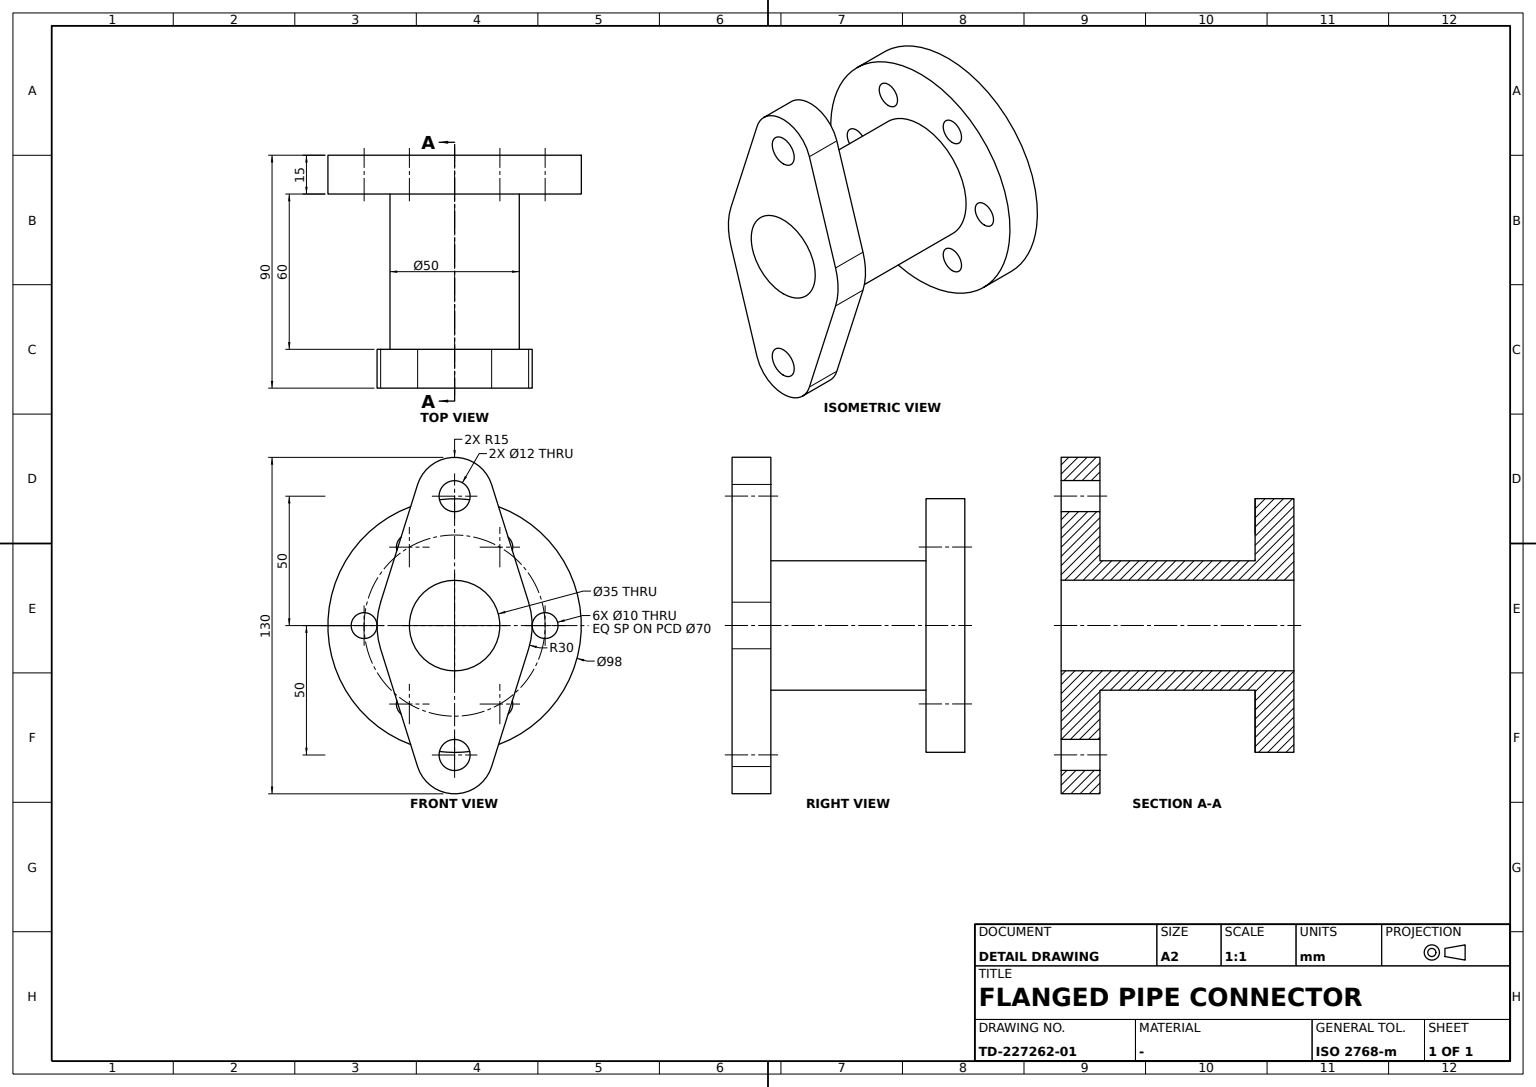
ISO-10303-21;
HEADER;
FILE_DESCRIPTION((''),'2;1');
FILE_NAME('','',(''),(''),'','','');
FILE_SCHEMA(('AUTOMOTIVE_DESIGN'));
ENDSEC;
DATA;
#1=APPLICATION_CONTEXT('');
#2=PRODUCT_CONTEXT('',#1,'mechanical');
#3=PRODUCT('','','',(#2));
#4=PRODUCT_DEFINITION_FORMATION('','',#3);
#5=PRODUCT_DEFINITION_CONTEXT('',#1,'design');
#6=PRODUCT_DEFINITION('','',#4,#5);
#7=PRODUCT_DEFINITION_SHAPE('','',#6);
#8=(LENGTH_UNIT()NAMED_UNIT(*)SI_UNIT(.MILLI.,.METRE.));
#9=(NAMED_UNIT(*)PLANE_ANGLE_UNIT()SI_UNIT($,.RADIAN.));
#10=(NAMED_UNIT(*)SI_UNIT($,.STERADIAN.)SOLID_ANGLE_UNIT());
#11=UNCERTAINTY_MEASURE_WITH_UNIT(LENGTH_MEASURE(0.005),#8,'distance_accuracy_value','');
#12=(GEOMETRIC_REPRESENTATION_CONTEXT(3)GLOBAL_UNCERTAINTY_ASSIGNED_CONTEXT((#11))GLOBAL_UNIT_ASSIGNED_CONTEXT((#8,#9,#10))REPRESENTATION_CONTEXT('',''));
#13=CARTESIAN_POINT('',(15.,0.,-25.));
#14=VERTEX_POINT('',#13);
#15=CARTESIAN_POINT('',(15.,0.,0.));
#16=DIRECTION('',(1.,0.,0.));
#17=DIRECTION('',(0.,0.,-1.));
#18=AXIS2_PLACEMENT_3D('',#15,#16,#17);
#19=CIRCLE('',#18,25.);
#20=EDGE_CURVE('',#14,#14,#19,.T.);
#21=ORIENTED_EDGE('',*,*,#20,.T.);
#22=EDGE_LOOP('',(#21));
#23=FACE_BOUND('',#22,.T.);
#24=CARTESIAN_POINT('',(75.,0.,-25.));
#25=VERTEX_POINT('',#24);
#26=CARTESIAN_POINT('',(75.,0.,0.));
#27=AXIS2_PLACEMENT_3D('',#26,#16,#17);
#28=CIRCLE('',#27,25.);
#29=EDGE_CURVE('',#25,#25,#28,.T.);
#30=ORIENTED_EDGE('',*,*,#29,.F.);
#31=EDGE_LOOP('',(#30));
#32=FACE_BOUND('',#31,.T.);
#33=CARTESIAN_POINT('',(45.,0.,0.));
#34=DIRECTION('',(0.,1.,0.));
#35=AXIS2_PLACEMENT_3D('',#33,#16,#34);
#36=CYLINDRICAL_SURFACE('',#35,25.);
#37=ADVANCED_FACE('',(#23,#32),#36,.T.);
#38=CARTESIAN_POINT('',(90.,0.,-56.));
#39=VERTEX_POINT('',#38);
#40=CARTESIAN_POINT('',(90.,0.,-50.));
#41=AXIS2_PLACEMENT_3D('',#40,#16,#17);
#42=CIRCLE('',#41,6.);
#43=EDGE_CURVE('',#39,#39,#42,.T.);
#44=ORIENTED_EDGE('',*,*,#43,.T.);
#45=EDGE_LOOP('',(#44));
#46=FACE_BOUND('',#45,.T.);
#47=CARTESIAN_POINT('',(75.,0.,-56.));
#48=VERTEX_POINT('',#47);
#49=CARTESIAN_POINT('',(75.,0.,-50.));
#50=AXIS2_PLACEMENT_3D('',#49,#16,#17);
#51=CIRCLE('',#50,6.);
#52=EDGE_CURVE('',#48,#48,#51,.T.);
#53=ORIENTED_EDGE('',*,*,#52,.F.);
#54=EDGE_LOOP('',(#53));
#55=FACE_BOUND('',#54,.T.);
#56=CARTESIAN_POINT('',(82.5,0.,-50.));
#57=AXIS2_PLACEMENT_3D('',#56,#16,#34);
#58=CYLINDRICAL_SURFACE('',#57,6.);
#59=ADVANCED_FACE('',(#46,#55),#58,.F.);
#60=CARTESIAN_POINT('',(0.,17.5,-35.310889));
#61=VERTEX_POINT('',#60);
#62=CARTESIAN_POINT('',(0.,17.5,-30.310889));
#63=AXIS2_PLACEMENT_3D('',#62,#16,#17);
#64=CIRCLE('',#63,5.);
#65=EDGE_CURVE('',#61,#61,#64,.T.);
#66=ORIENTED_EDGE('',*,*,#65,.F.);
#67=EDGE_LOOP('',(#66));
#68=FACE_BOUND('',#67,.T.);
#69=CARTESIAN_POINT('',(15.,17.5,-35.310889));
#70=VERTEX_POINT('',#69);
#71=CARTESIAN_POINT('',(15.,17.5,-30.310889));
#72=AXIS2_PLACEMENT_3D('',#71,#16,#17);
#73=CIRCLE('',#72,5.);
#74=EDGE_CURVE('',#70,#70,#73,.T.);
#75=ORIENTED_EDGE('',*,*,#74,.T.);
#76=EDGE_LOOP('',(#75));
#77=FACE_BOUND('',#76,.T.);
#78=CARTESIAN_POINT('',(7.5,17.5,-30.310889));
#79=AXIS2_PLACEMENT_3D('',#78,#16,#34);
#80=CYLINDRICAL_SURFACE('',#79,5.);
#81=ADVANCED_FACE('',(#68,#77),#80,.F.);
#82=CARTESIAN_POINT('',(15.,0.,-49.));
#83=VERTEX_POINT('',#82);
#84=CIRCLE('',#18,49.);
#85=EDGE_CURVE('',#83,#83,#84,.T.);
#86=ORIENTED_EDGE('',*,*,#85,.F.);
#87=EDGE_LOOP('',(#86));
#88=FACE_BOUND('',#87,.T.);
#89=CARTESIAN_POINT('',(0.,0.,-49.));
#90=VERTEX_POINT('',#89);
#91=CARTESIAN_POINT('',(0.,0.,0.));
#92=AXIS2_PLACEMENT_3D('',#91,#16,#17);
#93=CIRCLE('',#92,49.);
#94=EDGE_CURVE('',#90,#90,#93,.T.);
#95=ORIENTED_EDGE('',*,*,#94,.T.);
#96=EDGE_LOOP('',(#95));
#97=FACE_BOUND('',#96,.T.);
#98=CARTESIAN_POINT('',(7.5,0.,0.));
#99=AXIS2_PLACEMENT_3D('',#98,#16,#34);
#100=CYLINDRICAL_SURFACE('',#99,49.);
#101=ADVANCED_FACE('',(#88,#97),#100,.T.);
#102=CARTESIAN_POINT('',(75.,-28.618176,9.));
#103=VERTEX_POINT('',#102);
#104=CARTESIAN_POINT('',(90.,-28.618176,9.));
#105=VERTEX_POINT('',#104);
#106=CARTESIAN_POINT('',(82.5,-28.618176,9.));
#107=VECTOR('',#16,1000.);
#108=LINE('',#106,#107);
#109=EDGE_CURVE('',#103,#105,#108,.T.);
#110=ORIENTED_EDGE('',*,*,#109,.T.);
#111=CARTESIAN_POINT('',(90.,-14.309088,54.5));
#112=VERTEX_POINT('',#111);
#113=DIRECTION('',(0.,0.3,0.953939201));
#114=VECTOR('',#113,1000.);
#115=LINE('',#104,#114);
#116=EDGE_CURVE('',#105,#112,#115,.T.);
#117=ORIENTED_EDGE('',*,*,#116,.T.);
#118=CARTESIAN_POINT('',(75.,-14.309088,54.5));
#119=VERTEX_POINT('',#118);
#120=CARTESIAN_POINT('',(82.5,-14.309088,54.5));
#121=LINE('',#120,#107);
#122=EDGE_CURVE('',#119,#112,#121,.T.);
#123=ORIENTED_EDGE('',*,*,#122,.F.);
#124=LINE('',#102,#114);
#125=EDGE_CURVE('',#103,#119,#124,.T.);
#126=ORIENTED_EDGE('',*,*,#125,.F.);
#127=EDGE_LOOP('',(#110,#117,#123,#126));
#128=FACE_BOUND('',#127,.T.);
#129=DIRECTION('',(0.,0.953939201,-0.3));
#130=AXIS2_PLACEMENT_3D('',#102,#129,#113);
#131=PLANE('',#130);
#132=ADVANCED_FACE('',(#128),#131,.F.);
#133=CARTESIAN_POINT('',(75.,14.309088,-54.5));
#134=VERTEX_POINT('',#133);
#135=CARTESIAN_POINT('',(75.,28.618176,-9.));
#136=VERTEX_POINT('',#135);
#137=LINE('',#135,#114);
#138=EDGE_CURVE('',#134,#136,#137,.T.);
#139=ORIENTED_EDGE('',*,*,#138,.T.);
#140=CARTESIAN_POINT('',(90.,28.618176,-9.));
#141=VERTEX_POINT('',#140);
#142=CARTESIAN_POINT('',(82.5,28.618176,-9.));
#143=LINE('',#142,#107);
#144=EDGE_CURVE('',#136,#141,#143,.T.);
#145=ORIENTED_EDGE('',*,*,#144,.T.);
#146=CARTESIAN_POINT('',(90.,14.309088,-54.5));
#147=VERTEX_POINT('',#146);
#148=LINE('',#140,#114);
#149=EDGE_CURVE('',#147,#141,#148,.T.);
#150=ORIENTED_EDGE('',*,*,#149,.F.);
#151=CARTESIAN_POINT('',(82.5,14.309088,-54.5));
#152=LINE('',#151,#107);
#153=EDGE_CURVE('',#134,#147,#152,.T.);
#154=ORIENTED_EDGE('',*,*,#153,.F.);
#155=EDGE_LOOP('',(#139,#145,#150,#154));
#156=FACE_BOUND('',#155,.T.);
#157=AXIS2_PLACEMENT_3D('',#133,#129,#113);
#158=PLANE('',#157);
#159=ADVANCED_FACE('',(#156),#158,.T.);
#160=CARTESIAN_POINT('',(90.,14.309088,54.5));
#161=VERTEX_POINT('',#160);
#162=CARTESIAN_POINT('',(90.,28.618176,9.));
#163=VERTEX_POINT('',#162);
#164=DIRECTION('',(0.,0.3,-0.953939201));
#165=VECTOR('',#164,1000.);
#166=LINE('',#162,#165);
#167=EDGE_CURVE('',#161,#163,#166,.T.);
#168=ORIENTED_EDGE('',*,*,#167,.T.);
#169=CARTESIAN_POINT('',(75.,28.618176,9.));
#170=VERTEX_POINT('',#169);
#171=CARTESIAN_POINT('',(82.5,28.618176,9.));
#172=LINE('',#171,#107);
#173=EDGE_CURVE('',#170,#163,#172,.T.);
#174=ORIENTED_EDGE('',*,*,#173,.F.);
#175=CARTESIAN_POINT('',(75.,14.309088,54.5));
#176=VERTEX_POINT('',#175);
#177=LINE('',#169,#165);
#178=EDGE_CURVE('',#176,#170,#177,.T.);
#179=ORIENTED_EDGE('',*,*,#178,.F.);
#180=CARTESIAN_POINT('',(82.5,14.309088,54.5));
#181=LINE('',#180,#107);
#182=EDGE_CURVE('',#176,#161,#181,.T.);
#183=ORIENTED_EDGE('',*,*,#182,.T.);
#184=EDGE_LOOP('',(#168,#174,#179,#183));
#185=FACE_BOUND('',#184,.T.);
#186=DIRECTION('',(0.,-0.953939201,-0.3));
#187=AXIS2_PLACEMENT_3D('',#175,#186,#164);
#188=PLANE('',#187);
#189=ADVANCED_FACE('',(#185),#188,.F.);
#190=CARTESIAN_POINT('',(15.,-17.5,-35.310889));
#191=VERTEX_POINT('',#190);
#192=CARTESIAN_POINT('',(15.,-17.5,-30.310889));
#193=AXIS2_PLACEMENT_3D('',#192,#16,#17);
#194=CIRCLE('',#193,5.);
#195=EDGE_CURVE('',#191,#191,#194,.T.);
#196=ORIENTED_EDGE('',*,*,#195,.T.);
#197=EDGE_LOOP('',(#196));
#198=FACE_BOUND('',#197,.T.);
#199=CARTESIAN_POINT('',(0.,-17.5,-35.310889));
#200=VERTEX_POINT('',#199);
#201=CARTESIAN_POINT('',(0.,-17.5,-30.310889));
#202=AXIS2_PLACEMENT_3D('',#201,#16,#17);
#203=CIRCLE('',#202,5.);
#204=EDGE_CURVE('',#200,#200,#203,.T.);
#205=ORIENTED_EDGE('',*,*,#204,.F.);
#206=EDGE_LOOP('',(#205));
#207=FACE_BOUND('',#206,.T.);
#208=CARTESIAN_POINT('',(7.5,-17.5,-30.310889));
#209=AXIS2_PLACEMENT_3D('',#208,#16,#34);
#210=CYLINDRICAL_SURFACE('',#209,5.);
#211=ADVANCED_FACE('',(#198,#207),#210,.F.);
#212=CARTESIAN_POINT('',(90.,0.,-17.5));
#213=VERTEX_POINT('',#212);
#214=CARTESIAN_POINT('',(90.,0.,0.));
#215=AXIS2_PLACEMENT_3D('',#214,#16,#17);
#216=CIRCLE('',#215,17.5);
#217=EDGE_CURVE('',#213,#213,#216,.T.);
#218=ORIENTED_EDGE('',*,*,#217,.T.);
#219=EDGE_LOOP('',(#218));
#220=FACE_BOUND('',#219,.T.);
#221=CARTESIAN_POINT('',(0.,0.,-17.5));
#222=VERTEX_POINT('',#221);
#223=CIRCLE('',#92,17.5);
#224=EDGE_CURVE('',#222,#222,#223,.T.);
#225=ORIENTED_EDGE('',*,*,#224,.F.);
#226=EDGE_LOOP('',(#225));
#227=FACE_BOUND('',#226,.T.);
#228=CARTESIAN_POINT('',(44.34,0.,0.));
#229=AXIS2_PLACEMENT_3D('',#228,#16,#34);
#230=CYLINDRICAL_SURFACE('',#229,17.5);
#231=ADVANCED_FACE('',(#220,#227),#230,.F.);
#232=CARTESIAN_POINT('',(75.,0.,44.));
#233=VERTEX_POINT('',#232);
#234=CARTESIAN_POINT('',(75.,0.,50.));
#235=AXIS2_PLACEMENT_3D('',#234,#16,#17);
#236=CIRCLE('',#235,6.);
#237=EDGE_CURVE('',#233,#233,#236,.T.);
#238=ORIENTED_EDGE('',*,*,#237,.T.);
#239=EDGE_LOOP('',(#238));
#240=FACE_BOUND('',#239,.T.);
#241=ORIENTED_EDGE('',*,*,#125,.T.);
#242=CIRCLE('',#235,15.);
#243=EDGE_CURVE('',#176,#119,#242,.T.);
#244=ORIENTED_EDGE('',*,*,#243,.F.);
#245=ORIENTED_EDGE('',*,*,#178,.T.);
#246=CIRCLE('',#27,30.);
#247=EDGE_CURVE('',#136,#170,#246,.T.);
#248=ORIENTED_EDGE('',*,*,#247,.F.);
#249=ORIENTED_EDGE('',*,*,#138,.F.);
#250=CARTESIAN_POINT('',(75.,-14.309088,-54.5));
#251=VERTEX_POINT('',#250);
#252=CIRCLE('',#50,15.);
#253=EDGE_CURVE('',#251,#134,#252,.T.);
#254=ORIENTED_EDGE('',*,*,#253,.F.);
#255=CARTESIAN_POINT('',(75.,-28.618176,-9.));
#256=VERTEX_POINT('',#255);
#257=DIRECTION('',(0.,-0.3,0.953939201));
#258=VECTOR('',#257,1000.);
#259=LINE('',#255,#258);
#260=EDGE_CURVE('',#251,#256,#259,.T.);
#261=ORIENTED_EDGE('',*,*,#260,.T.);
#262=EDGE_CURVE('',#103,#256,#246,.T.);
#263=ORIENTED_EDGE('',*,*,#262,.F.);
#264=EDGE_LOOP('',(#241,#244,#245,#248,#249,#254,#261,#263));
#265=FACE_BOUND('',#264,.T.);
#266=ORIENTED_EDGE('',*,*,#52,.T.);
#267=EDGE_LOOP('',(#266));
#268=FACE_BOUND('',#267,.T.);
#269=ORIENTED_EDGE('',*,*,#29,.T.);
#270=EDGE_LOOP('',(#269));
#271=FACE_BOUND('',#270,.T.);
#272=AXIS2_PLACEMENT_3D('',#26,#16,#34);
#273=PLANE('',#272);
#274=ADVANCED_FACE('',(#240,#265,#268,#271),#273,.F.);
#275=CARTESIAN_POINT('',(0.,17.5,25.310889));
#276=VERTEX_POINT('',#275);
#277=CARTESIAN_POINT('',(0.,17.5,30.310889));
#278=AXIS2_PLACEMENT_3D('',#277,#16,#17);
#279=CIRCLE('',#278,5.);
#280=EDGE_CURVE('',#276,#276,#279,.T.);
#281=ORIENTED_EDGE('',*,*,#280,.F.);
#282=EDGE_LOOP('',(#281));
#283=FACE_BOUND('',#282,.T.);
#284=CARTESIAN_POINT('',(15.,17.5,25.310889));
#285=VERTEX_POINT('',#284);
#286=CARTESIAN_POINT('',(15.,17.5,30.310889));
#287=AXIS2_PLACEMENT_3D('',#286,#16,#17);
#288=CIRCLE('',#287,5.);
#289=EDGE_CURVE('',#285,#285,#288,.T.);
#290=ORIENTED_EDGE('',*,*,#289,.T.);
#291=EDGE_LOOP('',(#290));
#292=FACE_BOUND('',#291,.T.);
#293=CARTESIAN_POINT('',(7.5,17.5,30.310889));
#294=AXIS2_PLACEMENT_3D('',#293,#16,#34);
#295=CYLINDRICAL_SURFACE('',#294,5.);
#296=ADVANCED_FACE('',(#283,#292),#295,.F.);
#297=CARTESIAN_POINT('',(90.,-28.618176,-9.));
#298=VERTEX_POINT('',#297);
#299=CARTESIAN_POINT('',(82.5,-28.618176,-9.));
#300=LINE('',#299,#107);
#301=EDGE_CURVE('',#256,#298,#300,.T.);
#302=ORIENTED_EDGE('',*,*,#301,.T.);
#303=CIRCLE('',#215,30.);
#304=EDGE_CURVE('',#105,#298,#303,.T.);
#305=ORIENTED_EDGE('',*,*,#304,.F.);
#306=ORIENTED_EDGE('',*,*,#109,.F.);
#307=ORIENTED_EDGE('',*,*,#262,.T.);
#308=EDGE_LOOP('',(#302,#305,#306,#307));
#309=FACE_BOUND('',#308,.T.);
#310=CARTESIAN_POINT('',(82.5,0.,0.));
#311=AXIS2_PLACEMENT_3D('',#310,#16,#34);
#312=CYLINDRICAL_SURFACE('',#311,30.);
#313=ADVANCED_FACE('',(#309),#312,.T.);
#314=CARTESIAN_POINT('',(90.,-14.309088,-54.5));
#315=VERTEX_POINT('',#314);
#316=LINE('',#297,#258);
#317=EDGE_CURVE('',#315,#298,#316,.T.);
#318=ORIENTED_EDGE('',*,*,#317,.T.);
#319=ORIENTED_EDGE('',*,*,#301,.F.);
#320=ORIENTED_EDGE('',*,*,#260,.F.);
#321=CARTESIAN_POINT('',(82.5,-14.309088,-54.5));
#322=LINE('',#321,#107);
#323=EDGE_CURVE('',#251,#315,#322,.T.);
#324=ORIENTED_EDGE('',*,*,#323,.T.);
#325=EDGE_LOOP('',(#318,#319,#320,#324));
#326=FACE_BOUND('',#325,.T.);
#327=DIRECTION('',(0.,0.953939201,0.3));
#328=AXIS2_PLACEMENT_3D('',#250,#327,#257);
#329=PLANE('',#328);
#330=ADVANCED_FACE('',(#326),#329,.F.);
#331=CARTESIAN_POINT('',(90.,0.,50.));
#332=AXIS2_PLACEMENT_3D('',#331,#16,#17);
#333=CIRCLE('',#332,15.);
#334=EDGE_CURVE('',#161,#112,#333,.T.);
#335=ORIENTED_EDGE('',*,*,#334,.F.);
#336=ORIENTED_EDGE('',*,*,#182,.F.);
#337=ORIENTED_EDGE('',*,*,#243,.T.);
#338=ORIENTED_EDGE('',*,*,#122,.T.);
#339=EDGE_LOOP('',(#335,#336,#337,#338));
#340=FACE_BOUND('',#339,.T.);
#341=CARTESIAN_POINT('',(82.5,0.,50.));
#342=AXIS2_PLACEMENT_3D('',#341,#16,#34);
#343=CYLINDRICAL_SURFACE('',#342,15.);
#344=ADVANCED_FACE('',(#340),#343,.T.);
#345=CIRCLE('',#41,15.);
#346=EDGE_CURVE('',#315,#147,#345,.T.);
#347=ORIENTED_EDGE('',*,*,#346,.F.);
#348=ORIENTED_EDGE('',*,*,#323,.F.);
#349=ORIENTED_EDGE('',*,*,#253,.T.);
#350=ORIENTED_EDGE('',*,*,#153,.T.);
#351=EDGE_LOOP('',(#347,#348,#349,#350));
#352=FACE_BOUND('',#351,.T.);
#353=CYLINDRICAL_SURFACE('',#57,15.);
#354=ADVANCED_FACE('',(#352),#353,.T.);
#355=ORIENTED_EDGE('',*,*,#65,.T.);
#356=EDGE_LOOP('',(#355));
#357=FACE_BOUND('',#356,.T.);
#358=ORIENTED_EDGE('',*,*,#204,.T.);
#359=EDGE_LOOP('',(#358));
#360=FACE_BOUND('',#359,.T.);
#361=CARTESIAN_POINT('',(0.,-17.5,25.310889));
#362=VERTEX_POINT('',#361);
#363=CARTESIAN_POINT('',(0.,-17.5,30.310889));
#364=AXIS2_PLACEMENT_3D('',#363,#16,#17);
#365=CIRCLE('',#364,5.);
#366=EDGE_CURVE('',#362,#362,#365,.T.);
#367=ORIENTED_EDGE('',*,*,#366,.T.);
#368=EDGE_LOOP('',(#367));
#369=FACE_BOUND('',#368,.T.);
#370=CARTESIAN_POINT('',(0.,-35.,-5.));
#371=VERTEX_POINT('',#370);
#372=CARTESIAN_POINT('',(0.,-35.,0.));
#373=AXIS2_PLACEMENT_3D('',#372,#16,#17);
#374=CIRCLE('',#373,5.);
#375=EDGE_CURVE('',#371,#371,#374,.T.);
#376=ORIENTED_EDGE('',*,*,#375,.T.);
#377=EDGE_LOOP('',(#376));
#378=FACE_BOUND('',#377,.T.);
#379=ORIENTED_EDGE('',*,*,#224,.T.);
#380=EDGE_LOOP('',(#379));
#381=FACE_BOUND('',#380,.T.);
#382=CARTESIAN_POINT('',(0.,35.,-5.));
#383=VERTEX_POINT('',#382);
#384=CARTESIAN_POINT('',(0.,35.,0.));
#385=AXIS2_PLACEMENT_3D('',#384,#16,#17);
#386=CIRCLE('',#385,5.);
#387=EDGE_CURVE('',#383,#383,#386,.T.);
#388=ORIENTED_EDGE('',*,*,#387,.T.);
#389=EDGE_LOOP('',(#388));
#390=FACE_BOUND('',#389,.T.);
#391=ORIENTED_EDGE('',*,*,#94,.F.);
#392=EDGE_LOOP('',(#391));
#393=FACE_BOUND('',#392,.T.);
#394=ORIENTED_EDGE('',*,*,#280,.T.);
#395=EDGE_LOOP('',(#394));
#396=FACE_BOUND('',#395,.T.);
#397=AXIS2_PLACEMENT_3D('',#91,#16,#34);
#398=PLANE('',#397);
#399=ADVANCED_FACE('',(#357,#360,#369,#378,#381,#390,#393,#396),#398,.F.);
#400=ORIENTED_EDGE('',*,*,#144,.F.);
#401=ORIENTED_EDGE('',*,*,#247,.T.);
#402=ORIENTED_EDGE('',*,*,#173,.T.);
#403=EDGE_CURVE('',#141,#163,#303,.T.);
#404=ORIENTED_EDGE('',*,*,#403,.F.);
#405=EDGE_LOOP('',(#400,#401,#402,#404));
#406=FACE_BOUND('',#405,.T.);
#407=ADVANCED_FACE('',(#406),#312,.T.);
#408=ORIENTED_EDGE('',*,*,#346,.T.);
#409=ORIENTED_EDGE('',*,*,#149,.T.);
#410=ORIENTED_EDGE('',*,*,#403,.T.);
#411=ORIENTED_EDGE('',*,*,#167,.F.);
#412=ORIENTED_EDGE('',*,*,#334,.T.);
#413=ORIENTED_EDGE('',*,*,#116,.F.);
#414=ORIENTED_EDGE('',*,*,#304,.T.);
#415=ORIENTED_EDGE('',*,*,#317,.F.);
#416=EDGE_LOOP('',(#408,#409,#410,#411,#412,#413,#414,#415));
#417=FACE_BOUND('',#416,.T.);
#418=ORIENTED_EDGE('',*,*,#217,.F.);
#419=EDGE_LOOP('',(#418));
#420=FACE_BOUND('',#419,.T.);
#421=CARTESIAN_POINT('',(90.,0.,44.));
#422=VERTEX_POINT('',#421);
#423=CIRCLE('',#332,6.);
#424=EDGE_CURVE('',#422,#422,#423,.T.);
#425=ORIENTED_EDGE('',*,*,#424,.F.);
#426=EDGE_LOOP('',(#425));
#427=FACE_BOUND('',#426,.T.);
#428=ORIENTED_EDGE('',*,*,#43,.F.);
#429=EDGE_LOOP('',(#428));
#430=FACE_BOUND('',#429,.T.);
#431=AXIS2_PLACEMENT_3D('',#214,#16,#34);
#432=PLANE('',#431);
#433=ADVANCED_FACE('',(#417,#420,#427,#430),#432,.T.);
#434=CARTESIAN_POINT('',(15.,-35.,-5.));
#435=VERTEX_POINT('',#434);
#436=CARTESIAN_POINT('',(15.,-35.,0.));
#437=AXIS2_PLACEMENT_3D('',#436,#16,#17);
#438=CIRCLE('',#437,5.);
#439=EDGE_CURVE('',#435,#435,#438,.T.);
#440=ORIENTED_EDGE('',*,*,#439,.F.);
#441=EDGE_LOOP('',(#440));
#442=FACE_BOUND('',#441,.T.);
#443=ORIENTED_EDGE('',*,*,#289,.F.);
#444=EDGE_LOOP('',(#443));
#445=FACE_BOUND('',#444,.T.);
#446=CARTESIAN_POINT('',(15.,-17.5,25.310889));
#447=VERTEX_POINT('',#446);
#448=CARTESIAN_POINT('',(15.,-17.5,30.310889));
#449=AXIS2_PLACEMENT_3D('',#448,#16,#17);
#450=CIRCLE('',#449,5.);
#451=EDGE_CURVE('',#447,#447,#450,.T.);
#452=ORIENTED_EDGE('',*,*,#451,.F.);
#453=EDGE_LOOP('',(#452));
#454=FACE_BOUND('',#453,.T.);
#455=ORIENTED_EDGE('',*,*,#85,.T.);
#456=EDGE_LOOP('',(#455));
#457=FACE_BOUND('',#456,.T.);
#458=ORIENTED_EDGE('',*,*,#74,.F.);
#459=EDGE_LOOP('',(#458));
#460=FACE_BOUND('',#459,.T.);
#461=CARTESIAN_POINT('',(15.,35.,-5.));
#462=VERTEX_POINT('',#461);
#463=CARTESIAN_POINT('',(15.,35.,0.));
#464=AXIS2_PLACEMENT_3D('',#463,#16,#17);
#465=CIRCLE('',#464,5.);
#466=EDGE_CURVE('',#462,#462,#465,.T.);
#467=ORIENTED_EDGE('',*,*,#466,.F.);
#468=EDGE_LOOP('',(#467));
#469=FACE_BOUND('',#468,.T.);
#470=ORIENTED_EDGE('',*,*,#195,.F.);
#471=EDGE_LOOP('',(#470));
#472=FACE_BOUND('',#471,.T.);
#473=ORIENTED_EDGE('',*,*,#20,.F.);
#474=EDGE_LOOP('',(#473));
#475=FACE_BOUND('',#474,.T.);
#476=AXIS2_PLACEMENT_3D('',#15,#16,#34);
#477=PLANE('',#476);
#478=ADVANCED_FACE('',(#442,#445,#454,#457,#460,#469,#472,#475),#477,.T.);
#479=ORIENTED_EDGE('',*,*,#237,.F.);
#480=EDGE_LOOP('',(#479));
#481=FACE_BOUND('',#480,.T.);
#482=ORIENTED_EDGE('',*,*,#424,.T.);
#483=EDGE_LOOP('',(#482));
#484=FACE_BOUND('',#483,.T.);
#485=CYLINDRICAL_SURFACE('',#342,6.);
#486=ADVANCED_FACE('',(#481,#484),#485,.F.);
#487=ORIENTED_EDGE('',*,*,#451,.T.);
#488=EDGE_LOOP('',(#487));
#489=FACE_BOUND('',#488,.T.);
#490=ORIENTED_EDGE('',*,*,#366,.F.);
#491=EDGE_LOOP('',(#490));
#492=FACE_BOUND('',#491,.T.);
#493=CARTESIAN_POINT('',(7.5,-17.5,30.310889));
#494=AXIS2_PLACEMENT_3D('',#493,#16,#34);
#495=CYLINDRICAL_SURFACE('',#494,5.);
#496=ADVANCED_FACE('',(#489,#492),#495,.F.);
#497=ORIENTED_EDGE('',*,*,#466,.T.);
#498=EDGE_LOOP('',(#497));
#499=FACE_BOUND('',#498,.T.);
#500=ORIENTED_EDGE('',*,*,#387,.F.);
#501=EDGE_LOOP('',(#500));
#502=FACE_BOUND('',#501,.T.);
#503=CARTESIAN_POINT('',(7.5,35.,0.));
#504=AXIS2_PLACEMENT_3D('',#503,#16,#34);
#505=CYLINDRICAL_SURFACE('',#504,5.);
#506=ADVANCED_FACE('',(#499,#502),#505,.F.);
#507=ORIENTED_EDGE('',*,*,#375,.F.);
#508=EDGE_LOOP('',(#507));
#509=FACE_BOUND('',#508,.T.);
#510=ORIENTED_EDGE('',*,*,#439,.T.);
#511=EDGE_LOOP('',(#510));
#512=FACE_BOUND('',#511,.T.);
#513=CARTESIAN_POINT('',(7.5,-35.,0.));
#514=AXIS2_PLACEMENT_3D('',#513,#16,#34);
#515=CYLINDRICAL_SURFACE('',#514,5.);
#516=ADVANCED_FACE('',(#509,#512),#515,.F.);
#517=CLOSED_SHELL('',(#37,#59,#81,#101,#132,#159,#189,#211,#231,#274,#296,#313,#330,#344,#354,#399,#407,#433,#478,#486,#496,#506,#516));
#518=MANIFOLD_SOLID_BREP('',#517);
#519=ADVANCED_BREP_SHAPE_REPRESENTATION('',(#518),#12);
#520=SHAPE_DEFINITION_REPRESENTATION(#7,#519);
ENDSEC;
END-ISO-10303-21;
